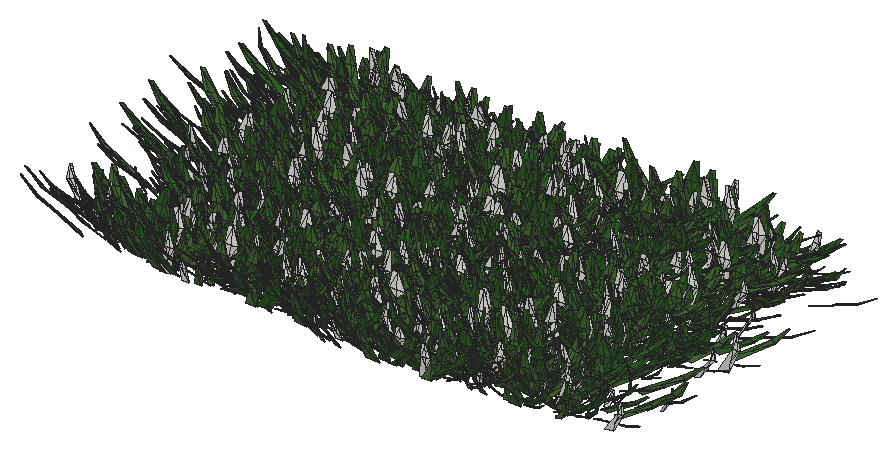
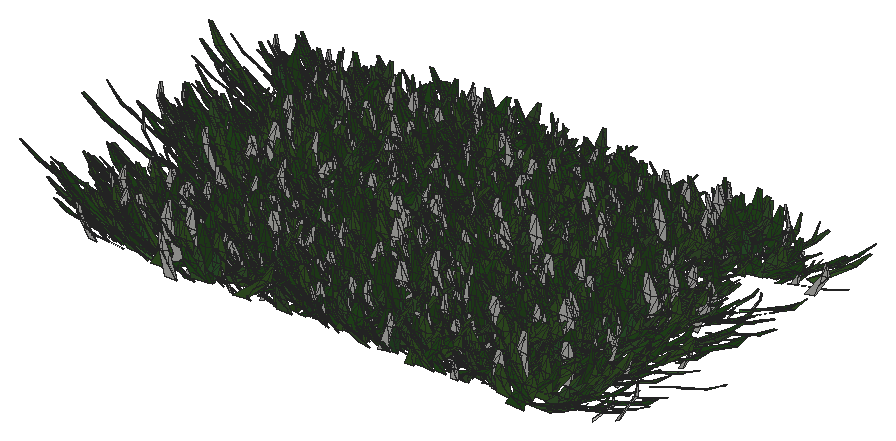
# SketchUp Ruby script. Lengths in inches.
U = 1.inch
M = Sketchup.active_model
def pt(a) = Geom::Point3d.new(a.map { |v| v * U })
def face(e, loops, mat)
  f = e.add_face(loops[0].map { |a| pt(a) })
  loops[1..].each { |l| e.add_face(l.map { |a| pt(a) }).erase! }
  f.material = f.back_material = mat if mat
  f
end
# faces: each face lists its corners as indices into pts; further lists are holes
def faces(e, pts, list, mat = nil) = list.each { |f| face(e, (f[0].is_a?(Array) ? f : [f]).map { |l| l.map { |i| pts[i] } }, mat) }
# xy, xz, yz: faces in a plane at the given z, y or x. An outline is a flat list of corners, or four numbers for a rectangle; further outlines are holes
def ring(l) = l.size == 4 ? [[l[0], l[1]], [l[2], l[1]], [l[2], l[3]], [l[0], l[3]]] : l.each_slice(2).to_a
def flat(e, list, mat, &to3) = list.each { |f| face(e, (f[0].is_a?(Array) ? f : [f]).map { |l| ring(l).map { |u, v| to3.(u, v) } }, mat) }
def xy(e, z, list, mat = nil) = flat(e, list, mat) { |x, y| [x, y, z] }
def xz(e, y, list, mat = nil) = flat(e, list, mat) { |x, z| [x, y, z] }
def yz(e, x, list, mat = nil) = flat(e, list, mat) { |y, z| [x, y, z] }
def lines(e, pts, list) = list.each { |a, b| e.add_line(pt(pts[a]), pt(pts[b])) }
# prism: a flat outline (further loops are holes) pulled along v
def prism(e, loops, v, mat = nil)
  f = face(e, loops, mat); d = Geom::Vector3d.new(v.map { |x| x * U })
  f.pushpull(f.normal.samedirection?(d) ? d.length : -d.length)
end
def box(e, o, s, mat = nil) = prism(e, [[o, [o[0] + s[0], o[1], o[2]], [o[0] + s[0], o[1] + s[1], o[2]], [o[0], o[1] + s[1], o[2]]]], [0, 0, s[2]], mat)
def at(x, y, z, deg = 0) = Geom::Transformation.translation(pt([x, y, z])) * Geom::Transformation.rotation(ORIGIN, Z_AXIS, deg.degrees)
def axes(o, x, y, z) = Geom::Transformation.new([*x, 0, *y, 0, *z, 0, *pt(o).to_a, 1])
def part(name) = M.definitions.add(name)
# library, detail: a bought-in or finely detailed component or shape, given as its bounding box
def library(name, o, s) = part(name).tap { |d| box(d.entities, o, s) }
def detail(e, o, s) = box(e.add_group.entities, o, s)
def put(e, d, t, mat = nil) = e.add_instance(d, t).tap { |i| i.material = mat if mat }
def group(e, t, mat = nil) = e.add_group.tap { |g| g.transformation = t; g.material = mat if mat }.entities
root = M.entities
M.materials.add("Material10").color = [48, 100, 38]
M.materials.add("Material3").color = [68, 110, 58]
M.materials.add("Material4").color = [48, 90, 38]
M.materials.add("Material5").color = [68, 110, 48]
M.materials.add("Material6").color = [48, 90, 48]
M.materials.add("Material7").color = [58, 110, 58]
M.materials.add("Material8").color = [58, 90, 38]
M.materials.add("Material9").color = [68, 100, 58]
c1 = part("grass00")
p = [[-0.6875,0.15,0],[-0.56,0.08,5.52],[-0.04,0.03,2.76],[0.48,-0.02,0],[0.35,-0.02,5.52],[-0.1,-0.14,5.52],
  [-0.12,0.65,8.37],[-0.42,0.65,8.37]]
faces(c1.entities,p,[[0,1,2,3],[3,2,4],[1,5,2],[5,4,2],[1,6,5],[4,5,6],[7,6,1]])
c2 = part("Group16\#1")
put(c2.entities,c1,axes([1.44,-0.61,-0.01],[0.05352,0.12609,0],[-0.10704,0.04543,0.07239],[0.06664,-0.02828,0.11628]),"Material6")
put(c2.entities,c1,axes([0.76,-0.15,-0.01],[0.04676,0.24062,0],[-0.23162,0.04501,0.06642],[0.0652,-0.01267,0.23595]),"Material3")
put(c2.entities,c1,axes([0.79,0.01,-0.01],[-0.00606,0.34651,0],[-0.34381,-0.00602,0.0432],[0.04319,0.00076,0.34386]))
put(c2.entities,c1,axes([1,0.23,-0.01],[-0.07192,0.31144,0],[-0.28722,-0.06632,0.1236],[0.12043,0.02781,0.29478]),"Material5")
put(c2.entities,c1,axes([1.66,0.77,-0.01],[-0.13828,0.29651,0],[-0.21551,-0.1005,0.22471],[0.20365,0.09498,0.23779]),"Material10")
put(c2.entities,c1,axes([0.6875,0.52,-0.01],[-0.18126,0.24051,0],[-0.22746,-0.17142,0.09788],[0.07817,0.05891,0.28481]),"Material5")
put(c2.entities,c1,axes([0.68,0.78,-0.01],[-0.215,0.18688,0],[-0.12385,-0.14248,0.21334],[0.13995,0.16101,0.18878]),"Material3")
put(c2.entities,c1,axes([0.56,1,-0.01],[-0.13756,0.07624,0],[-0.06159,-0.11112,0.0927],[0.04494,0.08108,0.12705]),"Material5")
put(c2.entities,c1,axes([0.2,0.64,-0.01],[-0.23729,0.07254,0],[-0.05711,-0.18681,0.153],[0.04473,0.14632,0.19535]),"Material10")
put(c2.entities,c1,axes([0.0625,0.72,-0.01],[-0.28874,0.02525,0],[-0.02179,-0.24916,0.14647],[0.01276,0.14591,0.25012]),"Material3")
put(c2.entities,c1,axes([-0.08,0.62,-0.01],[-0.34089,-0.04187,0],[0.03255,-0.26504,0.216],[-0.02633,0.21439,0.26703]),"Material10")
put(c2.entities,c1,axes([-0.34,0.98,-0.01],[-0.14314,-0.0493,0],[0.04397,-0.12769,0.06843],[-0.02228,0.0647,0.13505]),"Material10")
put(c2.entities,c1,axes([-0.87,1.45,-0.01],[-0.23488,-0.14114,0],[0.13761,-0.22901,0.06087],[-0.03135,0.05217,0.26717]))
put(c2.entities,c1,axes([-0.72,0.77,-0.01],[-0.14208,-0.13251,0],[0.07209,-0.0773,0.16301],[-0.11118,0.11922,0.1057]),"Material10")
put(c2.entities,c1,axes([-0.62,0.43,-0.01],[-0.14845,-0.21203,0],[0.18654,-0.13061,0.12304],[-0.10079,0.07057,0.22772]),"Material3")
put(c2.entities,c1,axes([-0.68,0.29,-0.01],[-0.13639,-0.32136,0],[0.31723,-0.13464,0.05579],[-0.05136,0.0218,0.34462]),"Material4")
put(c2.entities,c1,axes([-0.64,0.125,-0.01],[-0.0458,-0.23569,0],[0.22124,-0.043,0.08276],[-0.08124,0.01579,0.22538]),"Material7")
put(c2.entities,c1,axes([-1.6,-0.03,-0.01],[0.00576,-0.32897,0],[0.27526,0.00482,0.18018],[-0.18015,-0.00315,0.2753]),"Material5")
put(c2.entities,c1,axes([-1.36,-0.31,-0.01],[0.05718,-0.24765,0],[0.18172,0.04196,0.17267],[-0.16825,-0.03885,0.1865]),"Material10")
put(c2.entities,c1,axes([-1.54,-0.72,-0.01],[0.06537,-0.14017,0],[0.13555,0.06321,0.03939],[-0.0357,-0.01665,0.14956]))
put(c2.entities,c1,axes([-1.19,-0.9,-0.01],[0.09597,-0.12735,0],[0.11214,0.08451,0.07557],[-0.06035,-0.04548,0.14042]),"Material9")
put(c2.entities,c1,axes([-0.47,-0.54,-0.01],[0.11588,-0.10072,0],[0.0618,0.0711,0.12124],[-0.07953,-0.0915,0.0942]))
put(c2.entities,c1,axes([-0.47,-0.84,-0.01],[0.11927,-0.0661,0],[0.06603,0.11913,0.00646],[-0.00313,-0.00565,0.13621]),"Material5")
put(c2.entities,c1,axes([-0.38,-1.24,-0.01],[0.28037,-0.08571,0],[0.0618,0.20215,0.20315],[-0.05939,-0.19428,0.21139]),"Material9")
put(c2.entities,c1,axes([-0.06,-0.66,-0.01],[0.22719,-0.01987,0],[0.01247,0.14255,0.17758],[-0.01547,-0.17691,0.1431]),"Material8")
put(c2.entities,c1,axes([0.11,-0.89,-0.01],[0.14882,0.01828,0],[-0.01058,0.08611,0.12229],[0.01491,-0.12138,0.08676]),"Material6")
put(c2.entities,c1,axes([0.25,-0.72,-0.01],[0.20481,0.07053,0],[-0.06206,0.18022,0.10291],[0.03351,-0.0973,0.1906]),"Material6")
put(c2.entities,c1,axes([0.85,-1.42,-0.01],[0.16481,0.09904,0],[-0.09472,0.15762,0.05616],[0.02893,-0.04814,0.18389]),"Material5")
put(c2.entities,c1,axes([1.01,-1.09,-0.01],[0.21858,0.20385,0],[-0.17495,0.1876,0.15339],[0.10462,-0.11218,0.25652]),"Material10")
put(c2.entities,c1,axes([1.01,-0.71,-0.01],[0.08733,0.12473,0],[-0.06445,0.04512,0.13037],[0.1068,-0.07477,0.07867]),"Material6")
c3 = part("Group15\#1")
put(c3.entities,c2,at(0,0,0))
c4 = part("3darcstudiotree_grass00\#1")
put(c4.entities,c3,at(0,0,0))
put(root,c4,axes([845.39,924.125,0],[1.98106,1.05685,0],[-3.80639,0.44594,-0.0367],[-0.25209,0.02953,1.99296]))
put(root,c4,axes([847.04,895.56,0],[-3.60106,-0.04271,0],[0.19063,-1.00459,-0.03298],[0.01167,-0.06151,1.87797]))
put(root,c4,axes([847.21,911.86,0],[-3.73728,-0.2351,0],[0.93348,-0.92746,-0.02412],[0.03985,-0.03959,1.61843]))
put(root,c4,axes([847.64,916.41,0],[-3.21626,-0.41381,0],[2.3246,-1.12922,-0.00712],[0.01691,-0.00821,1.64666]))
put(root,c4,axes([847.07,917.69,0],[-3.61281,0.55884,0],[-2.43371,-0.98335,-0.03047],[-0.07699,-0.03111,1.38852]))
put(root,c4,axes([846,897.93,0],[3.58951,0.93345,0],[-2.76207,0.66383,-0.03508],[-0.16897,0.04061,1.59982]))
put(root,c4,axes([847.23,896.65,0],[2.4755,-0.8869,0],[3.51902,0.61389,-0.05108],[0.27994,0.04883,1.79238]))
put(root,c4,axes([846.81,921.11,0],[-1.7461,0.91224,0],[-4.28122,-0.51216,-0.03408],[-0.14069,-0.01683,1.35762]))
put(root,c4,axes([848.38,919.27,0],[-0.33514,-1.12345,0],[4.93469,-0.09201,-0.02024],[0.12034,-0.00224,1.84439]))
put(root,c4,axes([847.47,913.39,0],[3.73698,-0.82778,0],[3.1181,0.87978,-0.01442],[0.06211,0.01752,1.90876]))
put(root,c4,axes([847.1,910.33,0],[-2.06798,0.88983,0],[-4.26064,-0.61886,-0.00809],[-0.04346,-0.00631,1.91363]))
put(root,c4,axes([847.56,906.47,0],[3.50587,-0.21147,0],[1.00871,1.0452,-0.01591],[0.01836,0.01902,1.32206]))
put(root,c4,axes([848.33,907.28,0],[-2.9418,0.84861,0],[-3.1669,-0.68615,-0.03703],[-0.16978,-0.03678,1.58908]))
put(root,c4,axes([847.49,925.48,0],[1.17878,0.99592,0],[-4.61929,0.34171,-0.04809],[-0.20938,0.01549,1.36712]))
put(root,c4,axes([847.63,904.27,0],[4.48137,0.06994,0],[-0.29564,1.18401,-0.00965],[-0.00318,0.01276,1.57035]))
put(root,c4,axes([849.2,915.42,0],[3.67211,-0.34396,0],[1.33384,0.89,-0.02122],[0.05893,0.03932,1.88089]))
put(root,c4,axes([851.37,924.17,0],[-3.47348,-0.25295,0],[1.42263,-1.22094,-0.03129],[0.05076,-0.04356,1.8441]))
put(root,c4,axes([851.56,914.87,0],[-3.84564,-0.10505,0],[0.54072,-1.23711,-0.01667],[0.01042,-0.02384,1.79039]))
put(root,c4,axes([852.05,907.7,0],[-4.66165,0.25618,0],[-0.8902,-1.01241,-0.01858],[-0.02067,-0.02351,1.34303]))
put(root,c4,axes([852.55,898.35,0],[-2.97895,-0.70139,0],[3.1973,-0.84873,-0.03536],[0.14976,-0.03975,1.8008]))
put(root,c4,axes([851.42,911.17,0],[-1.07038,1.23184,0],[-4.14964,-0.22536,-0.03052],[-0.1562,-0.00848,1.38983]))
put(root,c4,axes([851.39,917.95,0],[-0.92876,0.98956,0],[-4.3525,-0.25532,-0.03302],[-0.17329,-0.01017,1.5061]))
put(root,c4,axes([852.87,897.51,0],[1.90431,-1.19182,0],[3.88687,0.38816,-0.05078],[0.31147,0.0311,1.72798]))
put(root,c4,axes([851.99,895.52,0],[1.39207,0.89707,0],[-3.84824,0.37323,-0.02781],[-0.15819,0.01534,1.57422]))
put(root,c4,axes([853.61,914.07,0],[1.63221,-0.89951,0],[4.40071,0.49908,-0.00454],[0.01782,0.00202,1.30224]))
put(root,c4,axes([852.27,902.88,0],[3.72343,0.03185,0],[-0.16951,1.23856,-0.02332],[-0.00466,0.03402,1.80921]))
put(root,c4,axes([852.53,922.46,0],[1.17856,0.89964,0],[-4.07228,0.33342,-0.00037],[-0.00182,0.00015,1.37352]))
put(root,c4,axes([854.4,909.22,0],[-5.01358,0.24268,0],[-0.96954,-1.25187,-0.01839],[-0.01653,-0.02135,1.50803]))
put(root,c4,axes([854.65,901,0],[-1.78221,-0.81561,0],[4.04221,-0.55204,-0.05959],[0.23708,-0.03238,1.30502]))
put(root,c4,axes([853.8,921.21,0],[1.94348,-0.80631,0],[3.13656,0.47251,-0.04784],[0.31182,0.04697,1.7418]))
put(root,c4,axes([854.8,925.49,0],[-0.42607,-0.90558,0],[3.98828,-0.11728,-0.01277],[0.06985,-0.00205,1.38207]))
put(root,c4,axes([853.21,919.97,0],[0.24379,1.1856,0],[-4.61569,0.05932,-0.0387],[-0.22912,0.00294,1.71236]))
put(root,c4,axes([853.02,911.96,0],[1.54067,1.02539,0],[-4.80438,0.45117,-0.05425],[-0.27305,0.02564,1.72469]))
put(root,c4,axes([854.05,899.83,0],[-1.78772,1.13511,0],[-3.81437,-0.37546,-0.00571],[-0.03781,-0.00372,1.8245]))
put(root,c4,axes([854.28,906.39,0],[-1.04195,1.21147,0],[-4.05734,-0.2181,-0.03186],[-0.23525,-0.01265,1.95913]))
put(root,c4,axes([855.25,917.15,0],[3.07334,0.62938,0],[-2.31014,0.70504,-0.00694],[-0.03076,0.00939,1.5947]))
put(root,c4,axes([855.49,905.03,0],[5.00659,0.06984,0],[-0.21528,0.96462,-0.03032],[-0.01077,0.04826,1.54015]))
put(root,c4,axes([858.24,904.54,0],[-2.38105,-0.91178,0],[4.30884,-0.70326,-0.04707],[0.17067,-0.02786,1.39282]))
put(root,c4,axes([857.85,898.43,0],[-3.6738,0.0712,0],[-0.31805,-1.02562,-0.03359],[-0.01978,-0.06378,1.95875]))
put(root,c4,axes([857.45,919.75,0],[3.57103,-0.64395,0],[2.64716,0.9175,-0.00659],[0.02668,0.00925,1.95827]))
put(root,c4,axes([857.23,895.91,0],[4.29662,-0.26643,0],[1.12646,1.13536,-0.04456],[0.05263,0.05304,1.43455]))
put(root,c4,axes([859.0625,916.46,0],[-3.55163,-0.42804,0],[1.6107,-0.8353,-0.00927],[0.03461,-0.01795,1.99366]))
put(root,c4,axes([859.66,902.82,0],[-1.0061,-0.89228,0],[4.92324,-0.34695,-0.01485],[0.08067,-0.00569,1.80381]))
put(root,c4,axes([858.88,912.07,0],[0.65893,-0.95794,0],[4.25403,0.18289,-0.05034],[0.326,0.01402,1.77282]))
put(root,c4,axes([858.18,897.01,0],[4.30831,-0.62309,0],[2.18452,0.94404,-0.042],[0.12053,0.05209,1.56273]))
put(root,c4,axes([859.84,921.01,0],[-1.67207,-0.91895,0],[3.50462,-0.39855,-0.03768],[0.25255,-0.02872,1.77164]))
put(root,c4,axes([858.85,924.76,0],[-1.13491,0.99621,0],[-4.4644,-0.31787,-0.05457],[-0.24954,-0.01777,1.37935]))
put(root,c4,axes([860.22,925.8,0],[-3.91405,-0.00229,0],[0.01024,-1.09429,-0.04252],[0.00062,-0.06673,1.71753]))
put(root,c4,axes([859.9,923.22,0],[1.60501,-1.19589,0],[4.41908,0.37068,-0.04434],[0.27906,0.02341,1.93394]))
put(root,c4,axes([858.62,910.04,0],[3.60857,0.48959,0],[-2.46007,1.13325,-0.00178],[-0.00354,0.00163,1.34491]))
put(root,c4,axes([860.7,901.1,0],[-4.32765,0.00867,0],[-0.03775,-1.17772,-0.00779],[-0.00036,-0.01131,1.71052]))
put(root,c4,axes([860.29,906.2,0],[2.90531,-0.67717,0],[3.51467,0.94245,-0.02398],[0.07004,0.01878,1.37951]))
put(root,c4,axes([859.375,917.73,0],[-0.09714,1.01662,0],[-4.47384,-0.02672,-0.0357],[-0.18312,-0.00109,1.43525]))
put(root,c4,axes([860.09,908.59,0],[-1.68892,1.07101,0],[-4.3391,-0.42766,-0.03242],[-0.20319,-0.02003,1.96368]))
put(root,c4,axes([861.03,899.9375,0],[1.59366,-0.94661,0],[3.67989,0.3872,-0.00467],[0.02447,0.00258,1.41828]))
put(root,c4,axes([861.55,907.23,0],[-4.44666,-0.20996,0],[0.93231,-1.23409,-0.03943],[0.03763,-0.04981,1.61444]))
put(root,c4,axes([859.89,915.35,0],[5.15116,-0.12991,0],[0.48402,1.19956,-0.01121],[0.00488,0.0121,1.30781]))
put(root,c4,axes([860.84,913.94,0],[4.97159,0.14622,0],[-0.54256,1.15298,-0.02625],[-0.02079,0.04418,1.96735]))
put(root,c4,axes([863.22,898.31,0],[-3.82917,-0.57908,0],[2.69029,-1.11185,-0.00291],[0.00714,-0.00295,1.54121]))
put(root,c4,axes([863.4,904.46,0],[1.08411,-0.99343,0],[4.41709,0.30127,-0.01691],[0.09138,0.00623,1.6028]))
put(root,c4,axes([863.5,920.9375,0],[2.20022,-0.75251,0],[4.00552,0.73197,-0.0361],[0.16943,0.03096,1.80295]))
put(root,c4,axes([863.78,914.15,0],[4.14217,-0.13896,0],[0.55231,1.029,-0.04419],[0.03401,0.06336,1.50171]))
put(root,c4,axes([863.66,895.66,0],[3.46429,0.31864,0],[-1.65951,1.12765,-0.05896],[-0.1317,0.08949,1.94308]))
put(root,c4,axes([865.53,916.92,0],[-4.66063,0.03187,0],[-0.11925,-1.09003,-0.04984],[-0.00747,-0.06831,1.49526]))
put(root,c4,axes([865.5,917.78,0],[0.72703,-1.03791,0],[5.00906,0.2193,-0.04237],[0.25355,0.0111,1.93074]))
put(root,c4,axes([864.9,912.61,0],[-2.37788,0.70827,0],[-3.16948,-0.66506,-0.02769],[-0.12287,-0.02578,1.49833]))
put(root,c4,axes([864.99,907.15,0],[-1.33257,1.11257,0],[-3.55566,-0.26617,-0.04102],[-0.28293,-0.02118,1.67021]))
put(root,c4,axes([865.59,906.23,0],[-3.55507,0.28812,0],[-1.24707,-0.96172,-0.02033],[-0.04772,-0.0368,1.92362]))
put(root,c4,axes([864.61,925.45,0],[4.13598,0.19347,0],[-0.75584,1.00989,-0.00485],[-0.0061,0.00815,1.75633]))
put(root,c4,axes([864.47,899.84,0],[0.77095,1.02886,0],[-4.76297,0.22306,-0.00799],[-0.0391,0.00183,1.50733]))
put(root,c4,axes([865.27,909.36,0],[4.78466,-0.38044,0],[1.18012,0.92761,-0.00335],[0.00607,0.00477,1.45436]))
put(root,c4,axes([867.09,896.65,0],[-4.81545,-0.2901,0],[1.06341,-1.10323,-0.03666],[0.0394,-0.04088,1.30149]))
put(root,c4,axes([867.42,901.3,0],[-3.36311,-0.90745,0],[3.5657,-0.82593,-0.02123],[0.07378,-0.01709,1.43939]))
put(root,c4,axes([865.82,919.72,0],[4.34926,-0.09263,0],[0.33262,0.97608,-0.01096],[0.00735,0.02158,1.93666]))
put(root,c4,axes([867.24,924.05,0],[1.03751,-0.98763,0],[4.08479,0.26819,-0.03356],[0.19811,0.01301,1.61101]))
put(root,c4,axes([866.13,903,0],[4.36652,-0.10456,0],[0.38952,1.01663,-0.02913],[0.02165,0.05651,1.9903]))
put(root,c4,axes([867.62,915.08,0],[0.12365,-1.27532,0],[4.95988,0.03006,-0.04883],[0.25094,0.00152,1.59403]))
put(root,c4,axes([865.8,910.47,0],[1.52464,0.86954,0],[-4.15594,0.45544,-0.01361],[-0.07039,0.00771,1.60179]))
put(root,c4,axes([866.65,922.54,0],[4.76541,-0.43818,0],[1.55968,1.06014,-0.01984],[0.0463,0.03147,1.90869]))
put(root,c4,axes([869.5,908.125,0],[-3.49123,-0.27922,0],[1.51464,-1.18364,-0.00535],[0.00882,-0.00689,1.67969]))
put(root,c4,axes([869.66,914.03,0],[0.13314,-1.12565,0],[4.81374,0.03558,-0.0158],[0.0905,0.00067,1.72451]))
put(root,c4,axes([869.95,900.18,0],[0.0625,-0.92457,0],[5.11457,0.02161,-0.02351],[0.11863,0.0005,1.61343]))
put(root,c4,axes([869.29,905.625,0],[2.8016,-0.76743,0],[3.52577,0.80446,-0.03913],[0.15024,0.03428,1.55084]))
put(root,c4,axes([870.03,918.01,0],[-5.10128,0.24176,0],[-0.82054,-1.08211,-0.04366],[-0.05047,-0.06656,1.70895]))
put(root,c4,axes([870.375,912.42,0],[-4.96044,-0.06591,0],[0.25075,-1.17948,-0.02618],[0.00816,-0.03838,1.73378]))
put(root,c4,axes([870.75,925.71,0],[-3.94461,-0.5014,0],[1.7984,-0.88427,-0.05096],[0.14967,-0.07359,1.60728]))
put(root,c4,axes([869.4,924.64,0],[3.7762,-0.18672,0],[0.72842,0.92072,-0.00259],[0.00364,0.0046,1.70099]))
put(root,c4,axes([869.75,921.5,0],[3.67314,-0.43874,0],[1.76522,0.92366,-0.01719],[0.04935,0.02582,1.70421]))
put(root,c4,axes([871.51,901.47,0],[-3.44755,-0.92992,0],[3.38069,-0.78334,-0.01903],[0.09302,-0.02155,1.91973]))
put(root,c4,axes([870.41,908.65,0],[-2.366,0.989,0],[-3.30831,-0.49466,-0.01081],[-0.05313,-0.00794,1.38013]))
put(root,c4,axes([869.93,910.7,0],[2.16605,0.76484,0],[-3.80323,0.67318,-0.06047],[-0.22732,0.04024,1.34144]))
put(root,c4,axes([870.875,904.7,0],[-1.89044,1.0999,0],[-3.63234,-0.39019,-0.02574],[-0.12693,-0.01363,1.32606]))
put(root,c4,axes([870.87,916.99,0],[3.25343,-0.44268,0],[1.93711,0.88978,-0.04084],[0.14968,0.06875,1.94165]))
put(root,c4,axes([872.65,919.8,0],[-2.99003,-0.56506,0],[2.79267,-0.92359,-0.03674],[0.12403,-0.04102,1.62045]))
put(root,c4,axes([872.65,898.06,0],[-4.96013,0.01619,0],[-0.06304,-1.20724,-0.02897],[-0.0018,-0.03442,1.4344]))
put(root,c4,axes([871.3,896,0],[3.481,0.74238,0],[-3.25262,0.95321,-0.05603],[-0.20851,0.06111,1.79617]))
put(root,c4,axes([872.79,903.14,0],[-3.23012,0.53983,0],[-2.03325,-0.76039,-0.00767],[-0.03049,-0.0114,1.63569]))
put(root,c4,axes([873.12,923.19,0],[1.70325,-1.05974,0],[4.66988,0.4691,-0.03894],[0.22464,0.02257,1.95573]))
put(root,c4,axes([872.95,915.56,0],[2.4144,-1.08588,0],[3.3917,0.47133,-0.02727],[0.14209,0.01975,1.44583]))
put(root,c4,axes([872.35,896.79,0],[4.57432,-0.02417,0],[0.10814,1.27933,-0.00824],[0.00087,0.0103,1.59977]))
put(root,c4,axes([872.8,894.36,0],[4.10387,0.33855,0],[-1.15114,0.87212,-0.0401],[-0.09251,0.07009,1.69032]))
put(root,c4,axes([875.4,919.95,0],[-4.98676,0.19311,0],[-0.7421,-1.19771,-0.03016],[-0.02479,-0.04002,1.62739]))
put(root,c4,axes([876.45,911,0],[-1.79404,-0.94481,0],[3.82512,-0.45395,-0.00409],[0.0193,-0.00229,1.3842]))
put(root,c4,axes([875.84,895.22,0],[-3.73442,0.23061,0],[-0.95038,-0.96187,-0.03348],[-0.04929,-0.04988,1.52035]))
put(root,c4,axes([876.3,911.72,0],[2.59296,-0.87117,0],[4.05566,0.75445,-0.00846],[0.02997,0.00558,1.39582]))
put(root,c4,axes([877.18,906.45,0],[-3.94716,-0.15767,0],[0.6625,-1.03659,-0.01241],[0.00983,-0.01538,1.31731]))
put(root,c4,axes([875.97,915.03,0],[4.34642,-0.40872,0],[1.45862,0.96946,-0.01237],[0.03108,0.02066,1.84855]))
put(root,c4,axes([877.62,897.99,0],[-4.3345,-0.18054,0],[0.62418,-0.93658,-0.01531],[0.0191,-0.02866,1.80136]))
put(root,c4,axes([877.46,900.96,0],[1.02924,-1.1219,0],[3.76479,0.21587,-0.013],[0.10318,0.00592,1.96601]))
put(root,c4,axes([877.91,903.17,0],[-1.06084,-1.17828,0],[4.37174,-0.246,-0.03143],[0.16722,-0.00941,1.52743]))
put(root,c4,axes([878.24,918.62,0],[-1.72294,-1.06651,0],[4.16754,-0.42079,-0.01424],[0.06745,-0.00681,1.43479]))
put(root,c4,axes([877.76,904.09,0],[-0.48134,-1.10906,0],[3.87122,-0.10501,-0.05057],[0.36681,-0.00995,1.77563]))
put(root,c4,axes([876.65,913.62,0],[3.37993,0.45978,0],[-1.93327,0.88823,-0.04213],[-0.10808,0.04966,1.35679]))
put(root,c4,axes([877.97,900.4,0],[3.21509,-0.82009,0],[3.01925,0.73979,-0.0131],[0.0637,0.01561,1.79861]))
put(root,c4,axes([878.9,920.66,0],[-3.80165,-0.22525,0],[1.19413,-1.25962,-0.00987],[0.01044,-0.01102,1.48448]))
put(root,c4,axes([876.91,909.07,0],[3.93668,0.7746,0],[-2.90323,0.92217,-0.01986],[-0.08093,0.02571,1.93312]))
put(root,c4,axes([877.81,897.12,0],[-0.79276,1.18933,0],[-3.59183,-0.14964,-0.00349],[-0.02047,-0.00085,1.35435]))
put(root,c4,axes([878.92,907.04,0],[2.16099,-1.18023,0],[3.73882,0.42786,-0.04178],[0.24002,0.02747,1.62381]))
put(root,c4,axes([877.98,916.18,0],[3.61999,0.64217,0],[-2.78348,0.98067,-0.05586],[-0.16431,0.05789,1.52805]))
put(root,c4,axes([879.82,926.3,0],[3.28078,-0.54762,0],[2.6685,0.99917,-0.03164],[0.11118,0.04163,1.90074]))
put(root,c4,axes([879.04,924.6,0],[1.88884,1.20061,0],[-4.32214,0.42498,-0.01805],[-0.11016,0.01083,1.90362]))
put(root,c4,axes([879.64,922.375,0],[4.87019,-0.36873,0],[1.38522,1.1435,-0.03542],[0.04951,0.04087,1.44036]))
put(root,c4,axes([881.57,910.73,0],[-3.20652,-0.59771,0],[2.76266,-0.9263,-0.01853],[0.05834,-0.01956,1.52144]))
put(root,c4,axes([881.89,918.74,0],[-4.04993,-0.77594,0],[2.93522,-0.9575,-0.01589],[0.04448,-0.01451,1.38765]))
put(root,c4,axes([881.53,922.62,0],[-4.54229,0.0918,0],[-0.30554,-0.94485,-0.02584],[-0.01532,-0.04736,1.74304]))
put(root,c4,axes([881.51,907.49,0],[3.29935,0.67285,0],[-2.48006,0.76006,-0.0073],[-0.03648,0.01118,1.93831]))
put(root,c4,axes([883.94,898.39,0],[-3.45897,-0.26737,0],[1.38281,-1.1181,-0.02785],[0.05102,-0.04126,1.81462]))
put(root,c4,axes([883.21,901.61,0],[-1.6569,0.8411,0],[-3.67968,-0.45304,-0.03193],[-0.19007,-0.0234,1.70102]))
put(root,c4,axes([884.45,906.05,0],[-4.11024,0.08918,0],[-0.31404,-0.9046,-0.03872],[-0.02635,-0.07591,1.78675]))
put(root,c4,axes([883.41,903.01,0],[3.52313,0.28357,0],[-1.27249,0.9881,-0.048],[-0.10422,0.08093,1.83855]))
put(root,c4,axes([885.78,913.95,0],[-1.14436,-0.88187,0],[4.48808,-0.364,-0.01227],[0.07282,-0.00591,1.83962]))
put(root,c4,axes([885.29,925.83,0],[1.53749,-0.92212,0],[4.0104,0.41792,-0.02113],[0.10884,0.01134,1.51549]))
put(root,c4,axes([883.71,919.65,0],[1.39417,1.1395,0],[-4.86141,0.37174,-0.03143],[-0.13527,0.01034,1.42994]))
put(root,c4,axes([884.5,914.64,0],[4.06384,-0.63322,0],[2.31994,0.93055,-0.04378],[0.15154,0.06078,1.79394]))
put(root,c4,axes([884.16,916.28,0],[3.66016,0.09208,0],[-0.4718,1.17207,-0.00091],[-0.00045,0.00113,1.45853]))
put(root,c4,axes([884.05,909.2,0],[0.81023,1.10626,0],[-4.8699,0.22292,-0.04305],[-0.25037,0.01146,1.82947]))
put(root,c4,axes([884.22,897.48,0],[3.47121,0.32425,0],[-1.57021,1.05061,-0.02415],[-0.05805,0.03884,1.92547]))
put(root,c4,axes([884.54,911.88,0],[0.63588,1.22934,0],[-4.27821,0.13831,-0.04685],[-0.28868,0.00933,1.67517]))
put(root,c4,axes([885.85,920.98,0],[1.12622,-0.91153,0],[3.70574,0.28616,-0.03395],[0.20191,0.01559,1.50895]))
put(root,c4,axes([884.78,895.83,0],[3.08399,0.48066,0],[-1.99021,0.79809,-0.0044],[-0.01295,0.00519,1.30779]))
put(root,c4,axes([884.79,924.09,0],[3.86594,0.83132,0],[-2.86233,0.83193,-0.04839],[-0.1699,0.04938,1.47711]))
put(root,c4,axes([884.9,899.65,0],[3.60165,0.48715,0],[-2.30784,1.06642,-0.00222],[-0.0056,0.00259,1.6055]))
put(root,c4,axes([885.45,904.64,0],[3.64912,0.26405,0],[-1.21989,1.05365,-0.02015],[-0.03346,0.0289,1.63787]))
put(root,c4,axes([888.16,907.73,0],[-2.66703,-0.80905,0],[2.89138,-0.59571,-0.03867],[0.19078,-0.03931,1.49724]))
put(root,c4,axes([888.72,910.39,0],[-3.90478,-0.61757,0],[2.54983,-1.00763,-0.01513],[0.04881,-0.01929,1.79885]))
put(root,c4,axes([888.59,897.46,0],[-3.22402,-0.42801,0],[2.1572,-1.01557,-0.05452],[0.12489,-0.05879,1.404]))
put(root,c4,axes([887.49,922.3125,0],[3.49835,-0.41383,0],[1.60405,0.84749,-0.01286],[0.03427,0.0181,1.45976]))
put(root,c4,axes([887.99,901.35,0],[-4.05846,0.5498,0],[-2.41739,-1.11529,-0.0133],[-0.0389,-0.01795,1.94738]))
